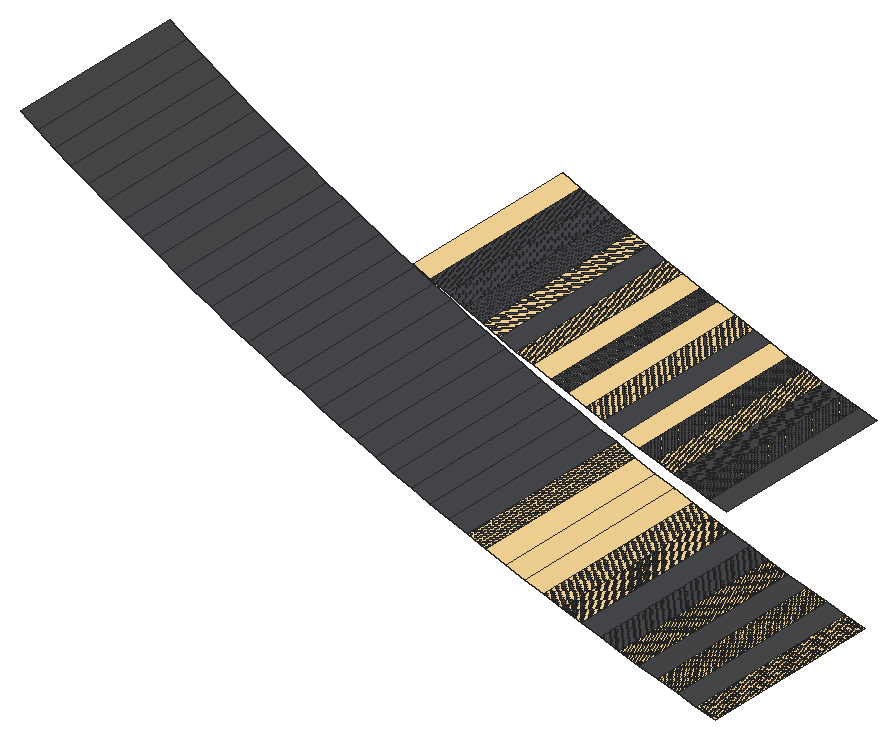
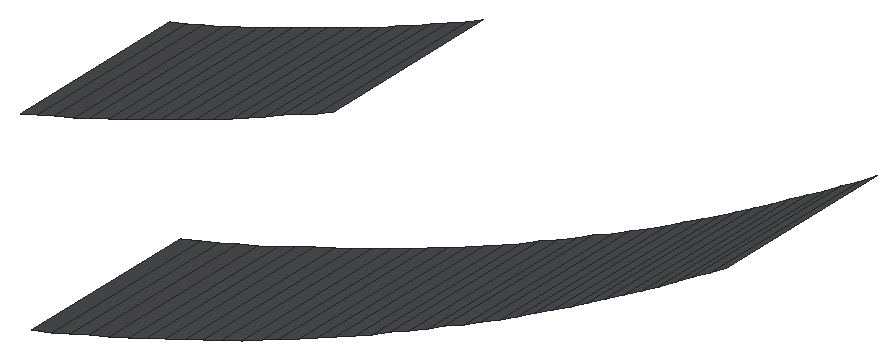
# SketchUp Ruby script. Lengths in inches.
U = 1.inch
M = Sketchup.active_model
def pt(a) = Geom::Point3d.new(a.map { |v| v * U })
def face(e, loops, mat)
  f = e.add_face(loops[0].map { |a| pt(a) })
  loops[1..].each { |l| e.add_face(l.map { |a| pt(a) }).erase! }
  f.material = f.back_material = mat if mat
  f
end
# faces: each face lists its corners as indices into pts; further lists are holes
def faces(e, pts, list, mat = nil) = list.each { |f| face(e, (f[0].is_a?(Array) ? f : [f]).map { |l| l.map { |i| pts[i] } }, mat) }
# xy, xz, yz: faces in a plane at the given z, y or x. An outline is a flat list of corners, or four numbers for a rectangle; further outlines are holes
def ring(l) = l.size == 4 ? [[l[0], l[1]], [l[2], l[1]], [l[2], l[3]], [l[0], l[3]]] : l.each_slice(2).to_a
def flat(e, list, mat, &to3) = list.each { |f| face(e, (f[0].is_a?(Array) ? f : [f]).map { |l| ring(l).map { |u, v| to3.(u, v) } }, mat) }
def xy(e, z, list, mat = nil) = flat(e, list, mat) { |x, y| [x, y, z] }
def xz(e, y, list, mat = nil) = flat(e, list, mat) { |x, z| [x, y, z] }
def yz(e, x, list, mat = nil) = flat(e, list, mat) { |y, z| [x, y, z] }
def lines(e, pts, list) = list.each { |a, b| e.add_line(pt(pts[a]), pt(pts[b])) }
# prism: a flat outline (further loops are holes) pulled along v
def prism(e, loops, v, mat = nil)
  f = face(e, loops, mat); d = Geom::Vector3d.new(v.map { |x| x * U })
  f.pushpull(f.normal.samedirection?(d) ? d.length : -d.length)
end
def box(e, o, s, mat = nil) = prism(e, [[o, [o[0] + s[0], o[1], o[2]], [o[0] + s[0], o[1] + s[1], o[2]], [o[0], o[1] + s[1], o[2]]]], [0, 0, s[2]], mat)
def at(x, y, z, deg = 0) = Geom::Transformation.translation(pt([x, y, z])) * Geom::Transformation.rotation(ORIGIN, Z_AXIS, deg.degrees)
def axes(o, x, y, z) = Geom::Transformation.new([*x, 0, *y, 0, *z, 0, *pt(o).to_a, 1])
def part(name) = M.definitions.add(name)
# library, detail: a bought-in or finely detailed component or shape, given as its bounding box
def library(name, o, s) = part(name).tap { |d| box(d.entities, o, s) }
def detail(e, o, s) = box(e.add_group.entities, o, s)
def put(e, d, t, mat = nil) = e.add_instance(d, t).tap { |i| i.material = mat if mat }
def group(e, t, mat = nil) = e.add_group.tap { |g| g.transformation = t; g.material = mat if mat }.entities
root = M.entities
M.materials.add("1432 AP 8245 TAR ROAD").color = [71, 72, 75]
M.materials.add("Outer Light").color = [251, 217, 152]
p = [[273.44,95.37,172.0625],[273.59,95.37,172.02],[273.59,96.87,172.02],[273.44,96.87,172.0625],[273.44,96.87,172.0625],[273.59,96.87,172.02],
  [273.59,95.37,172.02],[273.44,95.37,172.0625],[273.75,95.37,171.98],[273.75,96.87,171.98],[273.75,96.87,171.98],[273.75,95.37,171.98],
  [273.125,95.37,172.15],[273.28,95.37,172.11],[273.28,96.87,172.11],[273.125,96.87,172.15],[273.125,96.87,172.15],[273.28,96.87,172.11],
  [273.28,95.37,172.11],[273.125,95.37,172.15],[272.67,95.37,172.3],[272.82,95.37,172.25],[272.82,96.87,172.25],[272.67,96.87,172.3],
  [272.67,96.87,172.3],[272.82,96.87,172.25],[272.82,95.37,172.25],[272.67,95.37,172.3],[272.97,95.37,172.2],[272.97,96.87,172.2],
  [272.97,96.87,172.2],[272.97,95.37,172.2],[272.36,95.37,172.4],[272.51,95.37,172.35],[272.51,96.87,172.35],[272.36,96.87,172.4],
  [272.36,96.87,172.4],[272.51,96.87,172.35],[272.51,95.37,172.35],[272.36,95.37,172.4],[272.21,95.37,172.45],[272.21,96.87,172.45],
  [272.21,96.87,172.45],[272.21,95.37,172.45],[271.9,95.37,172.56],[272.06,95.37,172.5],[272.06,96.87,172.5],[271.9,96.87,172.56],
  [271.9,96.87,172.56],[272.06,96.87,172.5],[272.06,95.37,172.5],[271.9,95.37,172.56],[271.6,95.37,172.67],[271.75,95.37,172.62],
  [271.75,96.87,172.62],[271.6,96.87,172.67],[271.6,96.87,172.67],[271.75,96.87,172.62],[271.75,95.37,172.62],[271.6,95.37,172.67],
  [271.3,95.37,172.79],[271.45,95.37,172.73],[271.45,96.87,172.73],[271.3,96.87,172.79],[271.3,96.87,172.79],[271.45,96.87,172.73],
  [271.45,95.37,172.73],[271.3,95.37,172.79],[271.15,95.37,172.85],[271.15,96.87,172.85],[271.15,96.87,172.85],[271.15,95.37,172.85],
  [270.86,95.37,172.98],[271.01,95.37,172.91],[271.01,96.87,172.91],[270.86,96.87,172.98],[271.01,96.87,172.91],[271.01,95.37,172.91],
  [270.5625,95.37,173.11],[270.71,95.37,173.04],[270.71,96.87,173.04],[270.5625,96.87,173.11],[270.42,95.37,173.18],[270.42,96.87,173.18],
  [270.125,95.37,173.3125],[270.27,95.37,173.24],[270.27,96.87,173.24],[270.125,96.87,173.3125],[269.98,95.37,173.38],[269.98,96.87,173.38],
  [269.84,95.37,173.45],[269.84,96.87,173.45],[269.55,95.37,173.6],[269.69,95.37,173.53],[269.69,96.87,173.53],[269.55,96.87,173.6],
  [273.7,95.37,173.55],[273.56,95.37,173.59],[273.56,96.87,173.59],[273.7,96.87,173.55],[273.7,96.87,173.55],[273.56,96.87,173.59],
  [273.56,95.37,173.59],[273.7,95.37,173.55],[273.84,95.37,173.51],[273.84,96.87,173.51],[273.84,96.87,173.51],[273.84,95.37,173.51],
  [269.41,95.37,173.67],[269.41,96.87,173.67],[273.41,95.37,173.63],[273.27,95.37,173.68],[273.27,96.87,173.68],[273.41,96.87,173.63],
  [273.41,96.87,173.63],[273.27,96.87,173.68],[273.27,95.37,173.68],[273.41,95.37,173.63],[269.27,95.37,173.75],[269.27,96.87,173.75],
  [273.13,95.37,173.72],[272.99,95.37,173.77],[272.99,96.87,173.77],[273.13,96.87,173.72],[273.13,96.87,173.72],[272.99,96.87,173.77],
  [272.99,95.37,173.77],[273.13,95.37,173.72],[268.98,95.37,173.91],[269.125,95.37,173.83],[269.125,96.87,173.83],[268.98,96.87,173.91],
  [272.85,95.37,173.82],[272.7,95.37,173.87],[272.7,96.87,173.87],[272.85,96.87,173.82],[272.85,96.87,173.82],[272.7,96.87,173.87],
  [272.7,95.37,173.87],[272.85,95.37,173.82],[268.84,95.37,173.99],[268.84,96.87,173.99],[272.5625,95.37,173.92],[272.42,95.37,173.97],
  [272.42,96.87,173.97],[272.5625,96.87,173.92],[272.5625,96.87,173.92],[272.42,96.87,173.97],[272.42,95.37,173.97],[272.5625,95.37,173.92],
  [268.7,95.37,174.07],[268.7,96.87,174.07],[272.28,95.37,174.02],[272.14,95.37,174.07],[272.14,96.87,174.07],[272.28,96.87,174.02],
  [272.28,96.87,174.02],[272.14,96.87,174.07],[272.14,95.37,174.07],[272.28,95.37,174.02],[268.43,95.37,174.23],[268.56,95.37,174.15],
  [268.56,96.87,174.15],[268.43,96.87,174.23],[272.01,95.37,174.125],[271.87,95.37,174.18],[271.87,96.87,174.18],[272.01,96.87,174.125],
  [272.01,96.87,174.125],[271.87,96.87,174.18],[271.87,95.37,174.18],[272.01,95.37,174.125],[268.29,95.37,174.3125],[268.29,96.87,174.3125],
  [271.73,95.37,174.24],[271.59,95.37,174.3],[271.59,96.87,174.3],[271.73,96.87,174.24],[271.73,96.87,174.24],[271.59,96.87,174.3],
  [271.59,95.37,174.3],[271.73,95.37,174.24],[268.15,95.37,174.4],[268.15,96.87,174.4],[271.45,95.37,174.35],[271.45,96.87,174.35],
  [271.45,96.87,174.35],[271.45,95.37,174.35],[271.32,95.37,174.41],[271.32,96.87,174.41],[271.32,96.87,174.41],[271.32,95.37,174.41]]
faces(root,p,[[0,1,2,3],[1,8,9,2],[12,13,14,15],[13,0,3,14],[20,21,22,23],[21,28,29,22],[28,12,15,29],[32,33,34,35],
  [33,20,23,34],[40,32,35,41],[44,45,46,47],[45,40,41,46],[52,53,54,55],[53,44,47,54],[60,61,62,63],[61,52,55,62],
  [68,60,63,69],[72,73,74,75],[73,68,69,74],[78,79,80,81],[79,72,75,80],[82,78,81,83],[84,85,86,87],[85,82,83,86],
  [88,84,87,89],[90,88,89,91],[92,93,94,95],[93,90,91,94],[96,97,98,99],[104,96,99,105],[108,92,95,109],[110,111,112,113],
  [97,110,113,98],[118,108,109,119],[120,121,122,123],[111,120,123,112],[128,129,130,131],[129,118,119,130],[132,133,134,135],[121,132,135,122],
  [140,128,131,141],[142,143,144,145],[133,142,145,134],[150,140,141,151],[152,153,154,155],[143,152,155,144],[160,161,162,163],[161,150,151,162],
  [164,165,166,167],[153,164,167,154],[172,160,163,173],[174,175,176,177],[165,174,177,166],[182,172,173,183],[175,184,185,176],[184,188,189,185]],"1432 AP 8245 TAR ROAD")
faces(root,p,[[4,5,6,7],[5,10,11,6],[16,17,18,19],[17,4,7,18],[24,25,26,27],[25,30,31,26],[30,16,19,31],[36,37,38,39],
  [37,24,27,38],[42,36,39,43],[48,49,50,51],[49,42,43,50],[56,57,58,59],[57,48,51,58],[64,65,66,67],[65,56,59,66],
  [70,64,67,71],[76,70,71,77],[100,101,102,103],[106,100,103,107],[114,115,116,117],[101,114,117,102],[124,125,126,127],[115,124,127,116],
  [136,137,138,139],[125,136,139,126],[146,147,148,149],[137,146,149,138],[156,157,158,159],[147,156,159,148],[168,169,170,171],[157,168,171,158],
  [178,179,180,181],[169,178,181,170],[179,186,187,180],[186,190,191,187]],"Outer Light")
